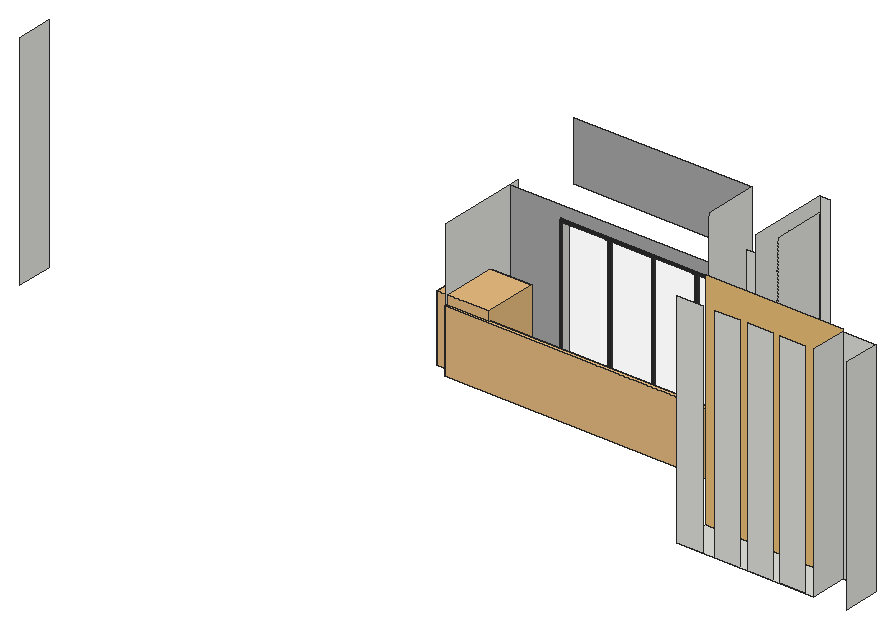
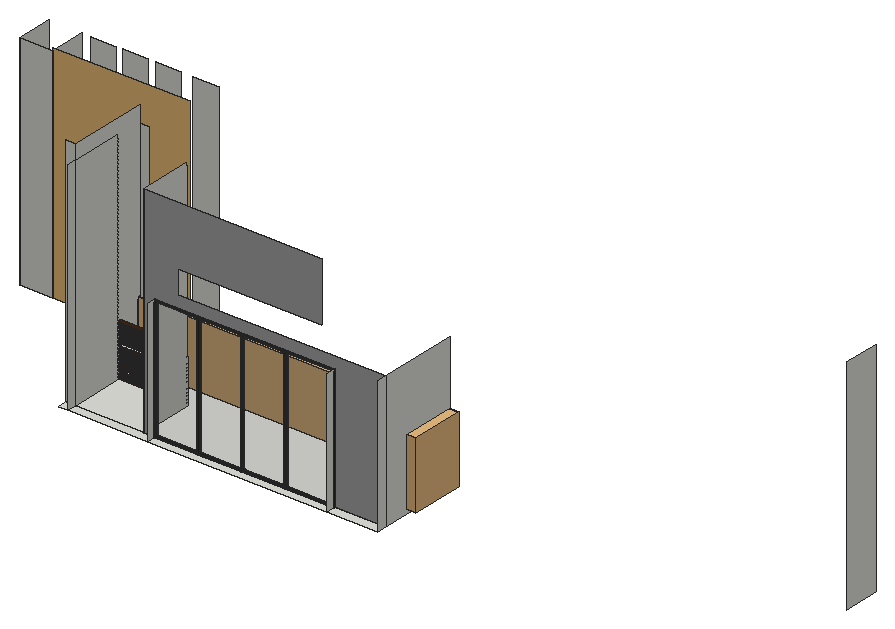
# SketchUp Ruby script. Lengths in inches.
U = 1.inch
M = Sketchup.active_model
def pt(a) = Geom::Point3d.new(a.map { |v| v * U })
def face(e, loops, mat)
  f = e.add_face(loops[0].map { |a| pt(a) })
  loops[1..].each { |l| e.add_face(l.map { |a| pt(a) }).erase! }
  f.material = f.back_material = mat if mat
  f
end
# faces: each face lists its corners as indices into pts; further lists are holes
def faces(e, pts, list, mat = nil) = list.each { |f| face(e, (f[0].is_a?(Array) ? f : [f]).map { |l| l.map { |i| pts[i] } }, mat) }
# xy, xz, yz: faces in a plane at the given z, y or x. An outline is a flat list of corners, or four numbers for a rectangle; further outlines are holes
def ring(l) = l.size == 4 ? [[l[0], l[1]], [l[2], l[1]], [l[2], l[3]], [l[0], l[3]]] : l.each_slice(2).to_a
def flat(e, list, mat, &to3) = list.each { |f| face(e, (f[0].is_a?(Array) ? f : [f]).map { |l| ring(l).map { |u, v| to3.(u, v) } }, mat) }
def xy(e, z, list, mat = nil) = flat(e, list, mat) { |x, y| [x, y, z] }
def xz(e, y, list, mat = nil) = flat(e, list, mat) { |x, z| [x, y, z] }
def yz(e, x, list, mat = nil) = flat(e, list, mat) { |y, z| [x, y, z] }
def lines(e, pts, list) = list.each { |a, b| e.add_line(pt(pts[a]), pt(pts[b])) }
# prism: a flat outline (further loops are holes) pulled along v
def prism(e, loops, v, mat = nil)
  f = face(e, loops, mat); d = Geom::Vector3d.new(v.map { |x| x * U })
  f.pushpull(f.normal.samedirection?(d) ? d.length : -d.length)
end
def box(e, o, s, mat = nil) = prism(e, [[o, [o[0] + s[0], o[1], o[2]], [o[0] + s[0], o[1] + s[1], o[2]], [o[0], o[1] + s[1], o[2]]]], [0, 0, s[2]], mat)
def at(x, y, z, deg = 0) = Geom::Transformation.translation(pt([x, y, z])) * Geom::Transformation.rotation(ORIGIN, Z_AXIS, deg.degrees)
def axes(o, x, y, z) = Geom::Transformation.new([*x, 0, *y, 0, *z, 0, *pt(o).to_a, 1])
def part(name) = M.definitions.add(name)
# library, detail: a bought-in or finely detailed component or shape, given as its bounding box
def library(name, o, s) = part(name).tap { |d| box(d.entities, o, s) }
def detail(e, o, s) = box(e.add_group.entities, o, s)
def put(e, d, t, mat = nil) = e.add_instance(d, t).tap { |i| i.material = mat if mat }
def group(e, t, mat = nil) = e.add_group.tap { |g| g.transformation = t; g.material = mat if mat }.entities
root = M.entities
M.materials.add("Glazing").color = [128, 128, 128]
M.materials["Glazing"].alpha = 0.05
M.materials.add("Powdercoating").color = [41, 44, 40]
M.materials.add("[Color M03]1").color = [170, 170, 170]
M.materials.add("[Wood OSB]1").color = [240, 195, 122]
M.materials.add("[Wood Veneer 01]").color = [96, 56, 29]
c1 = library("plant (1)",[-35.72,-28.42,0],[66.31,67.39,84.38])
c2 = part("Group\#15")
xy(c2.entities,0,[[0,-55.94,0.71,45.94]])
xy(c2.entities,0.2,[[0,-55.94,0.47,45.94],[0.47,45.94,0.71,46.42]])
xy(c2.entities,2.36,[[0.47,-55.94,0.71,46.42]])
xz(c2.entities,-55.94,[[0,0,0.71,0,0.71,2.36,0.47,2.36,0.47,0.2,0,0.2]])
xz(c2.entities,45.94,[[0,0,0.71,0.2]])
xz(c2.entities,46.42,[[0.47,0.2,0.71,2.36]])
yz(c2.entities,0,[[-55.94,0,45.94,0.2]])
yz(c2.entities,0.47,[[-55.94,0.2,46.42,2.36]])
yz(c2.entities,0.71,[[-55.94,0,45.94,0,45.94,0.2,46.42,0.2,46.42,2.36,-55.94,2.36]])
c3 = part("Group\#7")
xy(c3.entities,0,[[0,-59.09,0.71,45.94]])
xy(c3.entities,0.2,[[0,-59.09,0.47,45.94],[0.47,45.94,0.71,46.42]])
xy(c3.entities,2.36,[[0.47,-59.09,0.71,46.42]])
xz(c3.entities,-59.09,[[0,0,0.71,0,0.71,2.36,0.47,2.36,0.47,0.2,0,0.2]])
xz(c3.entities,45.94,[[0,0,0.71,0.2]])
xz(c3.entities,46.42,[[0.47,0.2,0.71,2.36]])
yz(c3.entities,0,[[-59.09,0,45.94,0.2]])
yz(c3.entities,0.47,[[-59.09,0.2,46.42,2.36]])
yz(c3.entities,0.71,[[-59.09,0,45.94,0,45.94,0.2,46.42,0.2,46.42,2.36,-59.09,2.36]])
c4 = part("Group\#16")
prism(c4.entities,[[[0.47,-56.18,0.2],[0,-56.18,0.2],[0,-56.18,0],[0.71,-56.18,0],[0.71,-56.18,2.36],[0.47,-56.18,2.36]]],[0,28.68,0])
c5 = part("Group\#10")
box(c5.entities,[-0.73,0,0],[27.99,0.55,102.05])
c6 = part("Group\#18")
xy(c6.entities,0,[[0.47,-56.18,0.47,-55.47,0,-55.47,0,-28.21,1.18,-28.21,1.18,-56.18]])
xy(c6.entities,0.2,[[0.71,-56.18,1.18,-28.21],[0,-55.47,0.47,-28.21],[0.47,-28.21,0.71,-27.74]])
xy(c6.entities,2.36,[[0.47,-56.18,0.71,-27.74]])
xz(c6.entities,-56.18,[[0.47,0,1.18,0,1.18,0.2,0.71,0.2,0.71,2.36,0.47,2.36]])
xz(c6.entities,-55.47,[[0,0,0.47,0.2]])
xz(c6.entities,-28.21,[[0,0,1.18,0.2]])
xz(c6.entities,-27.74,[[0.47,0.2,0.71,2.36]])
yz(c6.entities,0,[[-55.47,0,-28.21,0.2]])
yz(c6.entities,0.47,[[-56.18,0,-55.47,0.2],[-56.18,0.2,-27.74,2.36]])
yz(c6.entities,0.71,[[-56.18,0.2,-27.74,2.36]])
yz(c6.entities,1.18,[[-56.18,0,-28.21,0.2]])
c7 = part("Group\#34")
xy(c7.entities,0,[[-20.45,0,7.76,1.22]])
xy(c7.entities,0.06,[[-20.39,0.06,7.7,1.22]])
xy(c7.entities,0.47,[[-19.98,0,7.28,0.06]])
xy(c7.entities,101.89,[[-19.98,0,7.28,0.06]])
xy(c7.entities,102.3,[[-20.39,0.06,7.7,1.22]])
xy(c7.entities,102.36,[[-20.45,0,7.76,1.22]])
xz(c7.entities,0,[[[-20.45,0,7.76,102.36],[-19.98,0.47,7.28,101.89]]])
xz(c7.entities,0.06,[[[-20.39,0.06,7.7,102.3],[-19.98,0.47,7.28,101.89]]])
xz(c7.entities,1.22,[[[-20.45,0,7.76,102.36],[-20.39,0.06,7.7,102.3]]])
yz(c7.entities,-20.45,[[0,0,1.22,102.36]])
yz(c7.entities,-20.39,[[0.06,0.06,1.22,102.3]])
yz(c7.entities,-19.98,[[0,0.47,0.06,101.89]])
yz(c7.entities,7.28,[[0,0.47,0.06,101.89]])
yz(c7.entities,7.7,[[0.06,0.06,1.22,102.3]])
yz(c7.entities,7.76,[[0,0,1.22,102.36]])
c8 = part("Group\#6")
put(c8.entities,c2,axes([27.97,0,7.875],[1,0,0],[0,0,-1],[0,1,0]),"Powdercoating")
put(c8.entities,c3,axes([0.71,0,6.8],[-1,0,0],[0,0,-0.97687],[0,1,0]),"Powdercoating")
put(c8.entities,c4,axes([-27.5,0,-38.07],[0,0,-1],[-1,0,0],[0,1,0]),"Powdercoating")
put(c8.entities,c5,at(1.12,0.35,-38.39),"Glazing")
put(c8.entities,c6,axes([-27.5,0,63.35],[0,0,1],[-1,0,0],[0,1,0]),"Powdercoating")
put(c8.entities,c7,at(20.6875,1.0625,-38.54),"Powdercoating")
c9 = part("Component\#2")
put(c9.entities,c8,at(-1.18,4.5,38.86))
g1 = group(c9.entities,at(84.74,4.5,38.86))
put(g1,c2,axes([-27.97,0,7.875],[-1,0,0],[0,0,-1],[0,1,0]),"Powdercoating")
put(g1,c3,axes([-0.71,0,6.8],[1,0,0],[0,0,-0.97687],[0,1,0]),"Powdercoating")
put(g1,c4,axes([27.5,0,-38.07],[0,0,-1],[1,0,0],[0,1,0]),"Powdercoating")
put(g1,c5,axes([-1.12,0.35,-38.39],[-1,0,0],[0,1,0],[0,0,1]),"Glazing")
put(g1,c6,axes([27.5,0,63.35],[0,0,1],[1,0,0],[0,1,0]),"Powdercoating")
put(g1,c7,axes([-20.6875,1.0625,-38.54],[-1,0,0],[0,1,0],[0,0,1]),"Powdercoating")
g2 = group(c9.entities,at(56.0625,4.5,38.86))
put(g2,c2,axes([-27.97,0,7.875],[-1,0,0],[0,0,-1],[0,1,0]),"Powdercoating")
put(g2,c4,axes([27.5,0,-38.07],[0,0,-1],[1,0,0],[0,1,0]),"Powdercoating")
put(g2,c5,axes([-1.12,0.35,-38.39],[-1,0,0],[0,1,0],[0,0,1]),"Glazing")
put(g2,c6,axes([27.5,0,63.35],[0,0,1],[1,0,0],[0,1,0]),"Powdercoating")
put(g2,c7,axes([-20.6875,1.0625,-38.54],[-1,0,0],[0,1,0],[0,0,1]),"Powdercoating")
g3 = group(g2,at(-0.71,0,6.8),"Powdercoating")
xy(g3,-45.34,[[0.47,0.2,0.71,2.36]])
xy(g3,-44.88,[[0,0,0.71,0.2]])
xy(g3,57.73,[[0,0,0.71,0,0.71,2.36,0.47,2.36,0.47,0.2,0,0.2]])
xz(g3,0,[[0,-44.88,0.71,57.73]])
xz(g3,0.2,[[0.47,-45.34,0.71,-44.88],[0,-44.88,0.47,57.73]])
xz(g3,2.36,[[0.47,-45.34,0.71,57.73]])
yz(g3,0,[[0,-44.88,0.2,57.73]])
yz(g3,0.47,[[0.2,-45.34,2.36,57.73]])
yz(g3,0.71,[[0.2,-45.34,2.36,-45.34,2.36,57.73,0,57.73,0,-44.88,0.2,-44.88]])
put(c9.entities,c8,axes([-33.94,4.5,38.86],[1.14218,0,0],[0,1,0],[0,0,1]))
c10 = part("sliding door")
put(c10.entities,c9,at(0,-4.5,-0.08))
c11 = library("Glass Railing",[0,0,0],[139.5,4.76,42])
xy(root,191.19,[[1657.65,322.97,1831.09,368.59]])
xy(root,199,[[1276.37,433.78,1669.17,433.78,1669.17,465.95,1582.55,465.95,1582.55,534.98,1276.37,534.98],[1582.55,465.95,1669.17,534.98],[1276.37,534.98,1341.11,546.92],[1341.11,534.98,1568.55,546.92],[1568.55,534.98,1669.17,546.92],
  [1669.17,534.98,1681.11,546.92]])
xy(root,202.03,[[1582.55,465.95,1669.17,468.64]])
xy(root,202.9375,[[1582.55,465.95,1669.17,468.64]])
xy(root,205.97,[[1582.55,465.95,1669.17,468.64]])
xy(root,206.9375,[[1582.55,465.95,1669.17,468.64]])
xy(root,209.97,[[1582.55,465.95,1669.17,468.64]])
xy(root,211,[[1582.55,465.95,1669.17,468.64]])
xy(root,214.03,[[1582.55,465.95,1669.17,468.64]])
xy(root,215.0625,[[1582.55,465.95,1669.17,468.64]])
xy(root,218.09,[[1582.55,465.95,1669.17,468.64]])
xy(root,219.125,[[1582.55,465.95,1669.17,468.64]])
xy(root,222.16,[[1582.55,465.95,1669.17,468.64]])
xy(root,223.1875,[[1582.55,465.95,1669.17,468.64]])
xy(root,226.22,[[1582.55,465.95,1669.17,468.64]])
xy(root,227.25,[[1582.55,465.95,1669.17,468.64]])
xy(root,230.28,[[1582.55,465.95,1669.17,468.64]])
xy(root,231.3125,[[1582.55,465.95,1669.17,468.64]])
xy(root,234.34,[[1582.55,465.95,1669.17,468.64]])
xy(root,235.375,[[1582.55,465.95,1669.17,468.64]])
xy(root,238.41,[[1582.55,465.95,1669.17,468.64]])
xy(root,239.4375,[[1582.55,465.95,1669.17,468.64]])
xy(root,242.47,[[1582.55,465.95,1669.17,468.64]])
xy(root,243.5,[[1582.55,465.95,1669.17,468.64]])
xy(root,246.53,[[1582.55,465.95,1669.17,468.64]])
xy(root,247.5625,[[1582.55,465.95,1669.17,468.64]])
xy(root,250.59,[[1582.55,465.95,1669.17,468.64]])
xy(root,251.625,[[1582.55,465.95,1669.17,468.64]])
xy(root,254.66,[[1582.55,465.95,1669.17,468.64]])
xy(root,255.6875,[[1582.55,466.33,1669.17,468.64]])
xy(root,258.72,[[1582.55,466.33,1669.17,468.64]])
xy(root,259.75,[[1582.55,466.33,1669.17,468.64]])
xy(root,262.78,[[1582.55,466.33,1669.17,468.64]])
xy(root,263.8125,[[1582.55,466.33,1669.17,468.64]])
xz(root,322.97,[[1657.65,191.19,1689.86,471.94],[1705.34,191.19,1737.55,471.94],[1746.96,191.19,1779.17,471.94],[1787.59,191.19,1819.8,471.94]])
xz(root,368.59,[[1831.09,191.19,1872.84,471.94]])
xz(root,368.59,[[1657.65,191.19,1831.09,475.57]],"[Wood OSB]1")
xz(root,433.78,[[1657.65,199,1669.17,475.57]])
xz(root,465.95,[[1582.55,199,1669.17,202.03],[1582.55,202.9375,1669.17,205.97],[1582.55,206.9375,1669.17,209.97],[1582.55,211,1669.17,214.03],[1582.55,215.0625,1669.17,218.09],
  [1582.55,219.125,1669.17,222.16],[1582.55,223.1875,1669.17,226.22],[1582.55,227.25,1669.17,230.28],[1582.55,231.3125,1669.17,234.34],[1582.55,235.375,1669.17,238.41],
  [1582.55,239.4375,1669.17,242.47],[1582.55,243.5,1669.17,246.53],[1582.55,247.5625,1669.17,250.59],[1582.55,251.625,1669.17,254.66]],"[Wood Veneer 01]")
xz(root,466.33,[[1582.55,255.6875,1669.17,258.72],[1582.55,259.75,1669.17,262.78],[1582.55,263.8125,1669.17,266.84]],"[Wood Veneer 01]")
xz(root,468.64,[[1582.55,202.03,1669.17,202.9375],[1582.55,205.97,1669.17,206.9375],[1582.55,209.97,1669.17,211],[1582.55,214.03,1669.17,215.0625],[1582.55,218.09,1669.17,219.125],
  [1582.55,222.16,1669.17,223.1875],[1582.55,226.22,1669.17,227.25],[1582.55,230.28,1669.17,231.3125],[1582.55,234.34,1669.17,235.375],[1582.55,238.41,1669.17,239.4375],
  [1582.55,242.47,1669.17,243.5],[1582.55,246.53,1669.17,247.5625],[1582.55,250.59,1669.17,251.625],[1582.55,254.66,1669.17,255.6875],[1582.55,258.72,1669.17,259.75],
  [1582.55,262.78,1669.17,263.8125]])
xz(root,534.98,[[1669.17,199,1681.11,496.07]])
xz(root,534.98,[[1276.37,199,1341.11,199,1341.11,355.625,1568.55,355.625,1568.55,199,1582.55,199,1582.55,475.57,1356.97,475.57,1356.97,400,1539.31,400,1539.31,370.64,1276.37,370.64]],"[Color M03]1")
yz(root,824.53,[[322.97,191.19,368.59,471.94]])
yz(root,1276.37,[[433.78,199,534.98,370.64],[534.98,199,546.92,370.64]])
yz(root,1341.11,[[534.98,199,546.92,355.625]])
yz(root,1568.55,[[534.98,199,546.92,355.625]])
yz(root,1582.55,[[465.95,199,465.95,202.03,468.64,202.03,468.64,202.9375,465.95,202.9375,465.95,205.97,468.64,205.97,468.64,206.9375,465.95,206.9375,465.95,209.97,468.64,209.97,468.64,211,465.95,211,465.95,214.03,468.64,214.03,468.64,215.0625,465.95,215.0625,465.95,218.09,468.64,218.09,468.64,219.125,465.95,219.125,465.95,222.16,468.64,222.16,468.64,223.1875,465.95,223.1875,465.95,226.22,468.64,226.22,468.64,227.25,465.95,227.25,465.95,230.28,468.64,230.28,468.64,231.3125,465.95,231.3125,465.95,234.34,468.64,234.34,468.64,235.375,465.95,235.375,465.95,238.41,468.64,238.41,468.64,239.4375,465.95,239.4375,465.95,242.47,468.64,242.47,468.64,243.5,465.95,243.5,465.95,246.53,468.64,246.53,468.64,247.5625,465.95,247.5625,465.95,250.59,468.64,250.59,468.64,251.625,465.95,251.625,465.95,254.66,468.64,254.66,468.64,255.6875,466.33,255.6875,466.33,258.72,468.64,258.72,468.64,259.75,466.33,259.75,466.33,262.78,468.64,262.78,468.64,263.8125,466.33,263.8125,466.33,266.84,468.64,266.84,468.64,267.875,466.33,267.875,466.33,270.91,468.64,270.91,468.64,271.9375,466.33,271.9375,466.33,274.97,468.64,274.97,468.64,276,466.33,276,466.33,279.03,468.64,279.03,468.64,280.0625,466.33,280.0625,466.33,283.09,468.64,283.09,468.64,284.125,466.33,284.125,466.33,287.16,468.64,287.16,468.64,288.1875,466.33,288.1875,466.33,291.22,468.64,291.22,468.64,292.25,466.33,292.25,466.33,295.28,468.64,295.28,468.64,296.3125,466.33,296.3125,466.33,299.34,468.64,299.34,468.64,300.375,466.33,300.375,466.33,303.41,468.64,303.41,468.64,304.4375,466.33,304.4375,466.33,307.47,468.64,307.47,468.64,308.5,466.33,308.5,466.33,311.53,468.64,311.53,468.64,312.5625,466.33,312.5625,466.33,315.59,468.64,315.59,468.64,316.625,466.33,316.625,466.33,319.66,468.64,319.66,468.64,320.6875,466.33,320.6875,466.33,323.72,468.64,323.72,468.64,324.75,466.33,324.75,466.33,327.78,468.64,327.78,468.64,328.8125,466.33,328.8125,466.33,331.84,468.64,331.84,468.64,332.875,466.33,332.875,466.33,335.91,468.64,335.91,468.64,336.9375,466.33,336.9375,466.33,339.97,468.64,339.97,468.64,341,466.33,341,466.33,344.03,468.64,344.03,468.64,345.0625,466.33,345.0625,466.33,348.09,468.64,348.09,468.64,349.125,466.33,349.125,466.33,352.16,468.64,352.16,468.64,353.1875,466.33,353.1875,466.33,356.22,468.64,356.22,468.64,357.25,466.33,357.25,466.33,360.28,468.64,360.28,468.64,361.3125,466.33,361.3125,466.33,364.34,468.64,364.34,468.64,365.375,466.33,365.375,466.33,368.41,468.64,368.41,468.64,369.4375,466.33,369.4375,466.33,372.47,468.64,372.47,468.64,373.5,466.33,373.5,466.33,376.53,468.64,376.53,468.64,377.5625,466.33,377.5625,466.33,380.59,468.64,380.59,468.64,381.625,466.33,381.625,466.33,384.66,468.64,384.66,468.64,385.6875,466.33,385.6875,466.33,388.72,468.64,388.72,468.64,389.75,466.33,389.75,466.33,392.78,468.64,392.78,468.64,393.8125,466.33,393.8125,466.33,396.84,468.64,396.84,468.64,397.875,466.33,397.875,466.33,400.91,468.64,400.91,468.64,401.9375,466.33,401.9375,466.33,404.97,468.64,404.97,468.64,406,466.33,406,466.33,409.03,468.64,409.03,468.64,410.0625,466.33,410.0625,466.33,413.09,468.64,413.09,468.64,414.125,466.33,414.125,466.33,417.16,468.64,417.16,468.64,418.1875,466.33,418.1875,466.33,421.22,468.64,421.22,468.64,422.25,466.33,422.25,466.33,425.28,468.64,425.28,468.64,426.3125,466.33,426.3125,466.33,429.34,468.64,429.34,468.64,430.375,466.33,430.375,466.33,433.41,468.64,433.41,468.64,434.4375,466.33,434.4375,466.33,437.47,468.64,437.47,468.64,438.5,466.33,438.5,466.33,441.53,468.64,441.53,468.64,442.5625,466.33,442.5625,466.33,445.59,468.64,445.59,468.64,446.625,466.33,446.625,466.33,449.66,468.64,449.66,468.64,450.6875,466.33,450.6875,466.33,453.72,468.64,453.72,468.64,454.75,466.33,454.75,466.33,457.78,468.64,457.78,468.64,458.8125,466.33,458.8125,466.33,461.84,468.64,461.84,468.64,462.875,466.33,462.875,466.33,465.91,468.64,465.91,468.64,466.9375,466.33,466.9375,466.33,469.97,468.64,469.97,468.64,471,466.33,471,466.33,471.94,468.64,471.94,468.64,475.57,534.98,475.57,534.98,199]])
yz(root,1669.17,[[433.78,199,433.78,496.07,534.98,496.07,534.98,478.09,468.64,478.09,468.64,474.03,466.33,474.03,466.33,471,468.64,471,468.64,469.97,466.33,469.97,466.33,466.9375,468.64,466.9375,468.64,465.91,466.33,465.91,466.33,462.875,468.64,462.875,468.64,461.84,466.33,461.84,466.33,458.8125,468.64,458.8125,468.64,457.78,466.33,457.78,466.33,454.75,468.64,454.75,468.64,453.72,466.33,453.72,466.33,450.6875,468.64,450.6875,468.64,449.66,466.33,449.66,466.33,446.625,468.64,446.625,468.64,445.59,466.33,445.59,466.33,442.5625,468.64,442.5625,468.64,441.53,466.33,441.53,466.33,438.5,468.64,438.5,468.64,437.47,466.33,437.47,466.33,434.4375,468.64,434.4375,468.64,433.41,466.33,433.41,466.33,430.375,468.64,430.375,468.64,429.34,466.33,429.34,466.33,426.3125,468.64,426.3125,468.64,425.28,466.33,425.28,466.33,422.25,468.64,422.25,468.64,421.22,466.33,421.22,466.33,418.1875,468.64,418.1875,468.64,417.16,466.33,417.16,466.33,414.125,468.64,414.125,468.64,413.09,466.33,413.09,466.33,410.0625,468.64,410.0625,468.64,409.03,466.33,409.03,466.33,406,468.64,406,468.64,404.97,466.33,404.97,466.33,401.9375,468.64,401.9375,468.64,400.91,466.33,400.91,466.33,397.875,468.64,397.875,468.64,396.84,466.33,396.84,466.33,393.8125,468.64,393.8125,468.64,392.78,466.33,392.78,466.33,389.75,468.64,389.75,468.64,388.72,466.33,388.72,466.33,385.6875,468.64,385.6875,468.64,384.66,466.33,384.66,466.33,381.625,468.64,381.625,468.64,380.59,466.33,380.59,466.33,377.5625,468.64,377.5625,468.64,376.53,466.33,376.53,466.33,373.5,468.64,373.5,468.64,372.47,466.33,372.47,466.33,369.4375,468.64,369.4375,468.64,368.41,466.33,368.41,466.33,365.375,468.64,365.375,468.64,364.34,466.33,364.34,466.33,361.3125,468.64,361.3125,468.64,360.28,466.33,360.28,466.33,357.25,468.64,357.25,468.64,356.22,466.33,356.22,466.33,353.1875,468.64,353.1875,468.64,352.16,466.33,352.16,466.33,349.125,468.64,349.125,468.64,348.09,466.33,348.09,466.33,345.0625,468.64,345.0625,468.64,344.03,466.33,344.03,466.33,341,468.64,341,468.64,339.97,466.33,339.97,466.33,336.9375,468.64,336.9375,468.64,335.91,466.33,335.91,466.33,332.875,468.64,332.875,468.64,331.84,466.33,331.84,466.33,328.8125,468.64,328.8125,468.64,327.78,466.33,327.78,466.33,324.75,468.64,324.75,468.64,323.72,466.33,323.72,466.33,320.6875,468.64,320.6875,468.64,319.66,466.33,319.66,466.33,316.625,468.64,316.625,468.64,315.59,466.33,315.59,466.33,312.5625,468.64,312.5625,468.64,311.53,466.33,311.53,466.33,308.5,468.64,308.5,468.64,307.47,466.33,307.47,466.33,304.4375,468.64,304.4375,468.64,303.41,466.33,303.41,466.33,300.375,468.64,300.375,468.64,299.34,466.33,299.34,466.33,296.3125,468.64,296.3125,468.64,295.28,466.33,295.28,466.33,292.25,468.64,292.25,468.64,291.22,466.33,291.22,466.33,288.1875,468.64,288.1875,468.64,287.16,466.33,287.16,466.33,284.125,468.64,284.125,468.64,283.09,466.33,283.09,466.33,280.0625,468.64,280.0625,468.64,279.03,466.33,279.03,466.33,276,468.64,276,468.64,274.97,466.33,274.97,466.33,271.9375,468.64,271.9375,468.64,270.91,466.33,270.91,466.33,267.875,468.64,267.875,468.64,266.84,466.33,266.84,466.33,263.8125,468.64,263.8125,468.64,262.78,466.33,262.78,466.33,259.75,468.64,259.75,468.64,258.72,466.33,258.72,466.33,255.6875,468.64,255.6875,468.64,254.66,465.95,254.66,465.95,251.625,468.64,251.625,468.64,250.59,465.95,250.59,465.95,247.5625,468.64,247.5625,468.64,246.53,465.95,246.53,465.95,243.5,468.64,243.5,468.64,242.47,465.95,242.47,465.95,239.4375,468.64,239.4375,468.64,238.41,465.95,238.41,465.95,235.375,468.64,235.375,468.64,234.34,465.95,234.34,465.95,231.3125,468.64,231.3125,468.64,230.28,465.95,230.28,465.95,227.25,468.64,227.25,468.64,226.22,465.95,226.22,465.95,223.1875,468.64,223.1875,468.64,222.16,465.95,222.16,465.95,219.125,468.64,219.125,468.64,218.09,465.95,218.09,465.95,215.0625,468.64,215.0625,468.64,214.03,465.95,214.03,465.95,211,468.64,211,468.64,209.97,465.95,209.97,465.95,206.9375,468.64,206.9375,468.64,205.97,465.95,205.97,465.95,202.9375,468.64,202.9375,468.64,202.03,465.95,202.03,465.95,199],[465.95,199,465.95,202.03,468.64,202.03,468.64,202.9375,465.95,202.9375,465.95,205.97,468.64,205.97,468.64,206.9375,465.95,206.9375,465.95,209.97,468.64,209.97,468.64,211,465.95,211,465.95,214.03,468.64,214.03,468.64,215.0625,465.95,215.0625,465.95,218.09,468.64,218.09,468.64,219.125,465.95,219.125,465.95,222.16,468.64,222.16,468.64,223.1875,465.95,223.1875,465.95,226.22,468.64,226.22,468.64,227.25,465.95,227.25,465.95,230.28,468.64,230.28,468.64,231.3125,465.95,231.3125,465.95,234.34,468.64,234.34,468.64,235.375,465.95,235.375,465.95,238.41,468.64,238.41,468.64,239.4375,465.95,239.4375,465.95,242.47,468.64,242.47,468.64,243.5,465.95,243.5,465.95,246.53,468.64,246.53,468.64,247.5625,465.95,247.5625,465.95,250.59,468.64,250.59,468.64,251.625,465.95,251.625,465.95,254.66,468.64,254.66,468.64,255.6875,466.33,255.6875,466.33,258.72,468.64,258.72,468.64,259.75,466.33,259.75,466.33,262.78,468.64,262.78,468.64,263.8125,466.33,263.8125,466.33,266.84,468.64,266.84,468.64,267.875,466.33,267.875,466.33,270.91,468.64,270.91,468.64,271.9375,466.33,271.9375,466.33,274.97,468.64,274.97,468.64,276,466.33,276,466.33,279.03,468.64,279.03,468.64,280.0625,466.33,280.0625,466.33,283.09,468.64,283.09,468.64,284.125,466.33,284.125,466.33,287.16,468.64,287.16,468.64,288.1875,466.33,288.1875,466.33,291.22,468.64,291.22,468.64,292.25,466.33,292.25,466.33,295.28,468.64,295.28,468.64,296.3125,466.33,296.3125,466.33,299.34,468.64,299.34,468.64,300.375,466.33,300.375,466.33,303.41,468.64,303.41,468.64,304.4375,466.33,304.4375,466.33,307.47,468.64,307.47,468.64,308.5,466.33,308.5,466.33,311.53,468.64,311.53,468.64,312.5625,466.33,312.5625,466.33,315.59,468.64,315.59,468.64,316.625,466.33,316.625,466.33,319.66,468.64,319.66,468.64,320.6875,466.33,320.6875,466.33,323.72,468.64,323.72,468.64,324.75,466.33,324.75,466.33,327.78,468.64,327.78,468.64,328.8125,466.33,328.8125,466.33,331.84,468.64,331.84,468.64,332.875,466.33,332.875,466.33,335.91,468.64,335.91,468.64,336.9375,466.33,336.9375,466.33,339.97,468.64,339.97,468.64,341,466.33,341,466.33,344.03,468.64,344.03,468.64,345.0625,466.33,345.0625,466.33,348.09,468.64,348.09,468.64,349.125,466.33,349.125,466.33,352.16,468.64,352.16,468.64,353.1875,466.33,353.1875,466.33,356.22,468.64,356.22,468.64,357.25,466.33,357.25,466.33,360.28,468.64,360.28,468.64,361.3125,466.33,361.3125,466.33,364.34,468.64,364.34,468.64,365.375,466.33,365.375,466.33,368.41,468.64,368.41,468.64,369.4375,466.33,369.4375,466.33,372.47,468.64,372.47,468.64,373.5,466.33,373.5,466.33,376.53,468.64,376.53,468.64,377.5625,466.33,377.5625,466.33,380.59,468.64,380.59,468.64,381.625,466.33,381.625,466.33,384.66,468.64,384.66,468.64,385.6875,466.33,385.6875,466.33,388.72,468.64,388.72,468.64,389.75,466.33,389.75,466.33,392.78,468.64,392.78,468.64,393.8125,466.33,393.8125,466.33,396.84,468.64,396.84,468.64,397.875,466.33,397.875,466.33,400.91,468.64,400.91,468.64,401.9375,466.33,401.9375,466.33,404.97,468.64,404.97,468.64,406,466.33,406,466.33,409.03,468.64,409.03,468.64,410.0625,466.33,410.0625,466.33,413.09,468.64,413.09,468.64,414.125,466.33,414.125,466.33,417.16,468.64,417.16,468.64,418.1875,466.33,418.1875,466.33,421.22,468.64,421.22,468.64,422.25,466.33,422.25,466.33,425.28,468.64,425.28,468.64,426.3125,466.33,426.3125,466.33,429.34,468.64,429.34,468.64,430.375,466.33,430.375,466.33,433.41,468.64,433.41,468.64,434.4375,466.33,434.4375,466.33,437.47,468.64,437.47,468.64,438.5,466.33,438.5,466.33,441.53,468.64,441.53,468.64,442.5625,466.33,442.5625,466.33,445.59,468.64,445.59,468.64,446.625,466.33,446.625,466.33,449.66,468.64,449.66,468.64,450.6875,466.33,450.6875,466.33,453.72,468.64,453.72,468.64,454.75,466.33,454.75,466.33,457.78,468.64,457.78,468.64,458.8125,466.33,458.8125,466.33,461.84,468.64,461.84,468.64,462.875,466.33,462.875,466.33,465.91,468.64,465.91,468.64,466.9375,466.33,466.9375,466.33,469.97,468.64,469.97,468.64,471,466.33,471,466.33,474.03,468.64,474.03,468.64,478.09,534.98,478.09,534.98,199],[534.98,199,546.92,478.09]])
yz(root,1831.09,[[322.97,191.19,368.59,471.94]])
yz(root,1872.84,[[322.97,191.19,368.59,471.94]])
put(root,c1,at(1299.26,463.43,205.73))
put(root,c10,axes([1405.86,532.65,198.7],[1.9177,0,0],[0,1.51,0],[0,0,1.51]))
put(root,c11,axes([1276.37,431.36,198.94],[2.81576,0,0],[0,1,0],[0,0,1.9]))
